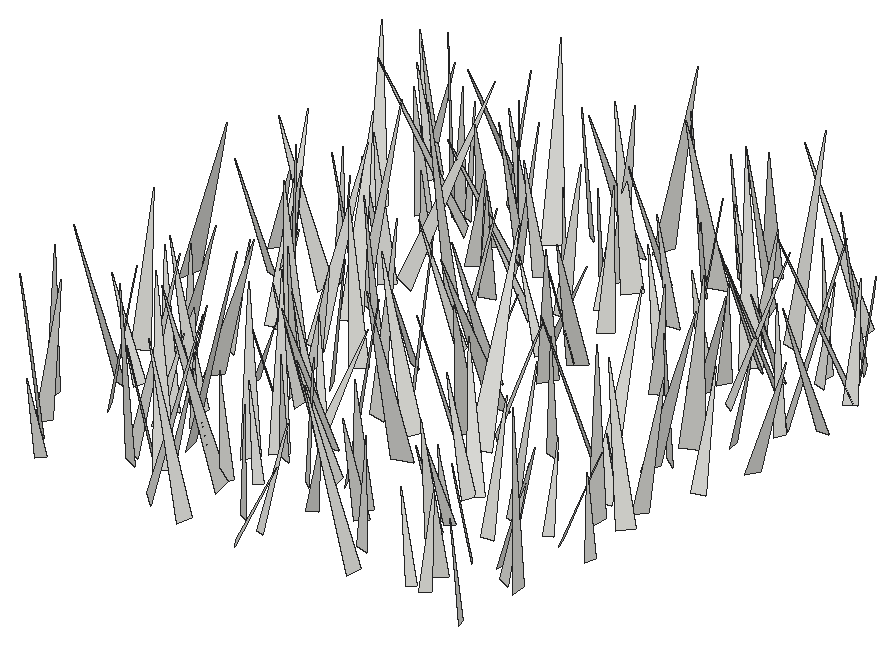
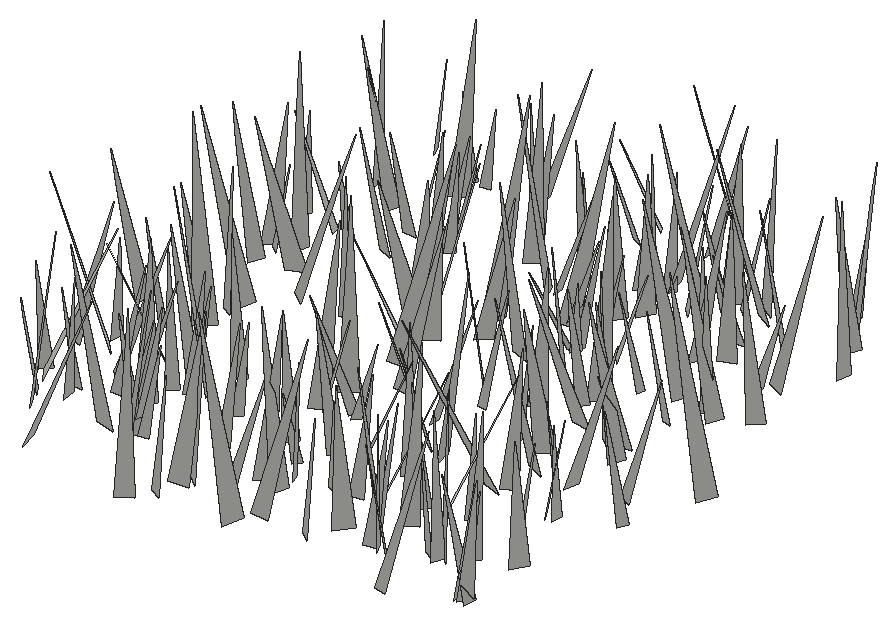
# SketchUp Ruby script. Lengths in inches.
U = 1.inch
M = Sketchup.active_model
def pt(a) = Geom::Point3d.new(a.map { |v| v * U })
def face(e, loops, mat)
  f = e.add_face(loops[0].map { |a| pt(a) })
  loops[1..].each { |l| e.add_face(l.map { |a| pt(a) }).erase! }
  f.material = f.back_material = mat if mat
  f
end
# faces: each face lists its corners as indices into pts; further lists are holes
def faces(e, pts, list, mat = nil) = list.each { |f| face(e, (f[0].is_a?(Array) ? f : [f]).map { |l| l.map { |i| pts[i] } }, mat) }
# xy, xz, yz: faces in a plane at the given z, y or x. An outline is a flat list of corners, or four numbers for a rectangle; further outlines are holes
def ring(l) = l.size == 4 ? [[l[0], l[1]], [l[2], l[1]], [l[2], l[3]], [l[0], l[3]]] : l.each_slice(2).to_a
def flat(e, list, mat, &to3) = list.each { |f| face(e, (f[0].is_a?(Array) ? f : [f]).map { |l| ring(l).map { |u, v| to3.(u, v) } }, mat) }
def xy(e, z, list, mat = nil) = flat(e, list, mat) { |x, y| [x, y, z] }
def xz(e, y, list, mat = nil) = flat(e, list, mat) { |x, z| [x, y, z] }
def yz(e, x, list, mat = nil) = flat(e, list, mat) { |y, z| [x, y, z] }
def lines(e, pts, list) = list.each { |a, b| e.add_line(pt(pts[a]), pt(pts[b])) }
# prism: a flat outline (further loops are holes) pulled along v
def prism(e, loops, v, mat = nil)
  f = face(e, loops, mat); d = Geom::Vector3d.new(v.map { |x| x * U })
  f.pushpull(f.normal.samedirection?(d) ? d.length : -d.length)
end
def box(e, o, s, mat = nil) = prism(e, [[o, [o[0] + s[0], o[1], o[2]], [o[0] + s[0], o[1] + s[1], o[2]], [o[0], o[1] + s[1], o[2]]]], [0, 0, s[2]], mat)
def at(x, y, z, deg = 0) = Geom::Transformation.translation(pt([x, y, z])) * Geom::Transformation.rotation(ORIGIN, Z_AXIS, deg.degrees)
def axes(o, x, y, z) = Geom::Transformation.new([*x, 0, *y, 0, *z, 0, *pt(o).to_a, 1])
def part(name) = M.definitions.add(name)
# library, detail: a bought-in or finely detailed component or shape, given as its bounding box
def library(name, o, s) = part(name).tap { |d| box(d.entities, o, s) }
def detail(e, o, s) = box(e.add_group.entities, o, s)
def put(e, d, t, mat = nil) = e.add_instance(d, t).tap { |i| i.material = mat if mat }
def group(e, t, mat = nil) = e.add_group.tap { |g| g.transformation = t; g.material = mat if mat }.entities
root = M.entities
c1 = part("fur_instance\#9")
p = [[0.8125,0,1.79],[0.67,-0.02,1.48],[0,-0.11,0],[0,0.11,0]]
faces(c1.entities,p,[[0,1,2,3]])
put(root,c1,axes([499.65,83.54,-21.66],[8.0282,-2.33719,0.44231],[-2.30718,-8.02996,-0.55383],[-0.57877,-0.40914,8.34313]))
put(root,c1,axes([503.88,99.4,-21.66],[-5.08982,4.44528,0.70369],[4.40622,5.13821,-0.58816],[0.91699,-0.01575,6.73207]))
put(root,c1,axes([503.84,105.55,-21.66],[3.17127,-3.30736,3.04126],[-3.82504,-3.9403,-0.2965],[-2.35731,1.94429,4.57249]))
put(root,c1,axes([501.91,90.21,-21.66],[3.6262,-2.26105,0.60128],[-2.31235,-3.63241,0.28605],[-0.35624,0.56255,4.26378]))
put(root,c1,axes([504.14,87.17,-21.66],[-1.82389,-4.57282,0.8897],[-4.65371,1.74485,-0.5721],[-0.21262,1.03617,4.88978]))
put(root,c1,axes([503.1,63.74,-21.66],[6.40054,-0.55178,2.21578],[-0.37829,-6.75939,-0.5905],[-2.25189,-0.43282,6.39709]))
put(root,c1,axes([504.66,105.33,-21.66],[-5.03296,-0.41167,1.23228],[-0.52474,5.15421,-0.42127],[1.18855,0.5323,5.03216]))
put(root,c1,axes([504.62,104.91,-21.66],[-3.50037,2.65675,1.28484],[2.86731,3.53339,0.50538],[0.69832,-1.19104,4.36526]))
put(root,c1,axes([503.78,72.875,-21.66],[3.27303,-4.65782,3.06275],[-5.40234,-3.52629,0.41046],[-1.37496,2.76738,5.67799]))
put(root,c1,axes([503.45,105.49,-21.66],[4.85484,-0.93426,0.93937],[-1.01134,-4.91828,0.33525],[-0.85583,0.51221,4.93253]))
put(root,c1,axes([505.83,68.11,-21.66],[-2.53564,-6.45433,1.27855],[-6.57975,2.48748,-0.49186],[0.00081,1.3699,6.91708]))
put(root,c1,axes([506.85,68.91,-21.66],[-3.73085,2.02538,0.45172],[2.07172,3.68874,0.57157],[0.11914,-0.71871,4.20651]))
put(root,c1,axes([504.86,60.56,-21.66],[5.24676,-2.59436,1.90695],[-2.83441,-5.4512,0.38233],[-1.5275,1.20389,5.84064]))
put(root,c1,axes([505.79,59.16,-21.66],[-4.21383,-5.23135,2.06774],[-5.35043,4.52497,0.54449],[1.7365,1.24763,6.69529]))
put(root,c1,axes([506.2,92.27,-21.66],[-3.76859,1.24193,1.36163],[1.17189,4.00702,-0.41131],[1.42236,-0.01087,3.94658]))
put(root,c1,axes([508.29,88.03,-21.66],[-6.63907,0.80935,0.83748],[0.8673,6.67065,0.42894],[0.7773,-0.53025,6.67446]))
put(root,c1,axes([507.12,92.4,-21.66],[-3.57369,-1.9669,1.0397],[-2.0892,3.64317,-0.28897],[0.76478,0.76131,4.06896]))
put(root,c1,axes([506.95,95.48,-21.66],[-3.35519,-0.75879,1.11745],[-0.66434,3.53232,0.40387],[1.17606,-0.1694,3.41613]))
put(root,c1,axes([507.09,100.62,-21.66],[4.37094,-3.26497,1.75227],[-3.26747,-4.6741,-0.55863],[-1.74761,0.57306,5.42707]))
put(root,c1,axes([507.36,73.87,-21.66],[1.49528,-4.80686,1.53266],[-5.04418,-1.45777,0.34917],[-0.10564,1.56838,5.02194]))
put(root,c1,axes([507.93,56.39,-21.66],[2.18541,-3.04998,0.78828],[-3.02604,-2.29919,-0.50659],[-0.87571,0.3334,3.71777]))
put(root,c1,axes([507.1875,65.12,-21.66],[5.44742,2.57642,1.57153],[2.74581,-5.57692,-0.37485],[-1.25227,-1.0208,6.0143]))
put(root,c1,axes([509.18,81.37,-21.66],[-1.39232,7.88876,0.40308],[7.89477,1.37627,0.33483],[-0.26016,-0.45487,8.00369]))
put(root,c1,axes([511.03,100.43,-21.66],[-6.73685,-3.71008,0.0403],[-3.70619,6.73292,0.28887],[0.17463,-0.23362,7.68547]))
put(root,c1,axes([508.9375,101.59,-21.66],[4.24793,5.0228,3.04998],[5.34423,-4.86703,0.57187],[-2.44337,-1.91294,6.55335]))
put(root,c1,axes([508.58,89.37,-21.66],[-3.28983,-1.54802,1.9149],[-2.00034,3.5437,-0.57187],[1.43591,1.38997,3.59058]))
put(root,c1,axes([506.34,74.3125,-21.66],[6.83641,-1.96558,0.32372],[-1.94381,-6.83529,-0.45298],[-0.43579,-0.34652,7.09893]))
put(root,c1,axes([508,83.29,-21.66],[5.45486,-2.53583,1.72286],[-2.73109,-5.61705,0.37948],[-1.39279,1.08278,6.00349]))
put(root,c1,axes([509.49,108.17,-21.66],[-2.17037,-5.72704,0.1674],[-5.69455,2.17595,0.61228],[0.63178,-0.0613,6.09382]))
put(root,c1,axes([509.23,81.25,-21.66],[1.43263,3.39143,0.32506],[3.34277,-1.46736,0.57677],[-0.65831,-0.07043,3.63615]))
put(root,c1,axes([508.81,76.67,-21.66],[1.57919,4.13225,1.33364],[4.34025,-1.54395,-0.35548],[-0.12772,-1.37428,4.40942]))
put(root,c1,axes([509,102.22,-21.66],[5.28351,-1.61661,1.62366],[-1.56193,-5.52709,-0.42043],[-1.67632,0.05465,5.50927]))
put(root,c1,axes([510,101.99,-21.66],[1.76175,3.91399,1.38102],[4.01071,-1.99148,0.5277],[-1.06803,-1.02224,4.25965]))
put(root,c1,axes([510.33,81.68,-21.66],[4.06784,5.47307,2.7985],[5.78633,-4.54195,0.47187],[-2.07475,-1.93641,6.80288]))
put(root,c1,axes([510.95,67.15,-21.66],[-2.98056,5.41129,1.99239],[5.72855,3.03527,0.32601],[0.65987,-1.90801,6.16924]))
put(root,c1,axes([511.4,91.1,-21.66],[-3.51075,4.42455,2.16586],[4.8357,3.60279,0.47842],[0.94002,-2.00904,5.62789]))
put(root,c1,axes([510.89,96.15,-21.66],[3.12862,-2.29976,0.97047],[-2.27,-3.26853,-0.42753],[-1.03819,0.21622,3.85932]))
put(root,c1,axes([512.72,68.39,-21.66],[-6.49588,1.72746,1.45223],[1.82521,6.62397,0.28488],[1.32729,-0.65455,6.71561]))
put(root,c1,axes([511.2,105.04,-21.66],[3.52114,3.87417,1.40413],[3.91467,-3.72163,0.45161],[-1.28689,-0.72073,5.21571]))
put(root,c1,axes([510.625,69.375,-21.66],[3.65523,2.01923,0.98653],[2.16689,-3.66612,-0.52479],[-0.59594,-0.94526,4.14277]))
put(root,c1,axes([512.76,85.38,-21.66],[-3.64093,6.72533,0.73654],[6.73348,3.68347,-0.34805],[0.65778,-0.48058,7.63972]))
put(root,c1,axes([511.72,87.85,-21.66],[2.95959,7.19025,1.54721],[7.29869,-3.07695,0.338],[-0.90704,-1.29822,7.76818]))
put(root,c1,axes([511.7,64.71,-21.66],[0.71871,3.7725,0.80138],[3.83913,-0.62217,-0.51422],[0.36739,-0.87844,3.80576]))
put(root,c1,axes([510.1,73.28,-21.66],[6.42408,-3.63909,0.41323],[-3.66082,-6.40525,0.50369],[-0.11006,0.64215,7.36601]))
put(root,c1,axes([513.28,59.77,-21.66],[2.89079,5.81329,3.19782],[6.3896,-3.37876,0.3661],[-1.787,-2.67707,6.48205]))
put(root,c1,axes([512.63,60.88,-21.66],[3.66563,6.83822,1.35122],[6.90712,-3.76874,0.33492],[-0.93742,-1.02919,7.75151]))
put(root,c1,axes([513.17,80.79,-21.66],[1.15921,7.66569,0.40932],[7.66684,-1.17697,0.3294],[-0.3873,-0.35503,7.74584]))
put(root,c1,axes([513.36,103.47,-21.66],[-4.21315,-2.34987,2.26772],[-2.4638,4.71684,0.31027],[2.14339,0.80291,4.81418]))
put(root,c1,axes([513.99,103.6,-21.66],[1.70929,-4.46495,1.67991],[-4.63149,-1.98085,-0.55231],[-1.1433,1.34907,4.74893]))
put(root,c1,axes([514.54,60.92,-21.66],[-2.99975,-3.60869,1.08185],[-3.74003,3.01886,-0.30041],[0.45307,1.02732,4.68304]))
put(root,c1,axes([512.39,91.81,-21.66],[3.274,7.7332,0.0389],[7.72076,-3.26624,-0.49451],[0.44025,-0.22856,8.38313]))
put(root,c1,axes([513.9375,66.23,-21.66],[0.22689,-3.51122,0.97081],[-3.62685,-0.12635,0.39066],[0.3422,0.98893,3.49679]))
put(root,c1,axes([512.95,74.34,-21.66],[3.6641,-0.22277,0.06955],[-0.2117,-3.63329,-0.48425],[-0.09821,-0.47926,3.63879]))
put(root,c1,axes([514.47,77.14,-21.66],[-4.81324,5.46383,3.73935],[6.29264,5.21276,0.48307],[2.05886,-3.15867,7.26549]))
put(root,c1,axes([515.17,85.24,-21.66],[-5.00491,-0.78513,1.46412],[-0.94309,5.16869,-0.45214],[1.36772,0.69095,5.0459]))
put(root,c1,axes([515.02,101.43,-21.66],[4.42222,0.57042,2.59632],[0.96066,-5.04183,-0.52855],[-2.47858,-0.93641,4.42741]))
put(root,c1,axes([513.71,99.57,-21.66],[4.30968,-5.09044,0.61484],[-5.06109,-4.35201,-0.55619],[-0.82219,0.10671,6.64655]))
put(root,c1,axes([515.89,60.39,-21.66],[-4.29093,5.93832,1.73067],[6.14946,4.32229,0.41585],[0.66564,-1.65078,7.31456]))
put(root,c1,axes([517.29,98.32,-21.66],[-5.15654,-2.89646,0.02201],[-2.88562,5.14083,0.47427],[0.2514,-0.40276,5.89529]))
put(root,c1,axes([514.44,96.9375,-21.66],[3.18493,-3.37138,0.77047],[-3.44968,-3.17103,0.3845],[-0.24394,0.82581,4.62191]))
put(root,c1,axes([514.95,78.4,-21.66],[2.82245,-3.27125,1.23973],[-3.47956,-2.78972,0.56063],[-0.36142,1.31172,4.28404]))
put(root,c1,axes([516.98,102.84,-21.66],[-5.31707,5.30249,0.96243],[5.27581,5.39738,-0.58989],[1.09932,-0.2564,7.48596]))
put(root,c1,axes([517.2,71.79,-21.66],[-2.83398,-2.56318,0.53676],[-2.6174,2.79801,-0.45803],[0.08496,0.70049,3.79362]))
put(root,c1,axes([516.24,74.73,-21.66],[5.75232,0.0292,2.58276],[0.25276,-6.28131,-0.49192],[-2.57052,-0.55229,5.73133]))
put(root,c1,axes([515.87,61.21,-21.66],[3.90442,0.1948,1.09665],[0.0575,-4.02752,0.51071],[-1.11233,0.47558,3.87577]))
put(root,c1,axes([517.37,80.45,-21.66],[-3.57367,4.96866,1.72232],[5.21894,3.60663,0.42422],[0.64547,-1.65218,6.10563]))
put(root,c1,axes([517.49,73.7,-21.66],[-4.79801,0.15244,1.14259],[0.25589,4.91001,0.4195],[1.12396,-0.46714,4.78206]))
put(root,c1,axes([517.96,90.46,-21.66],[-7.87878,-1.52664,2.20407],[-1.70967,8.13085,-0.47967],[2.06533,0.90687,8.01097]))
put(root,c1,axes([515.21,64.2,-21.66],[7.84011,2.17766,1.89393],[2.14429,-8.06482,0.39652],[-1.93163,-0.114,8.12726]))
put(root,c1,axes([517.49,63.48,-21.66],[-3.40896,-3.60182,1.17644],[-3.63778,3.55381,0.3393],[1.06005,0.61272,4.94762]))
put(root,c1,axes([516.77,99.27,-21.66],[3.29579,4.51514,1.8086],[4.80118,-3.36974,-0.33663],[-0.7786,-1.66678,5.57991]))
put(root,c1,axes([518.54,105.25,-21.66],[2.49829,3.83803,2.30798],[4.11646,-3.0089,0.54773],[-1.76409,-1.58579,4.54664]))
put(root,c1,axes([517.51,77.24,-21.66],[4.70905,2.28139,1.77217],[2.5251,-4.89691,-0.40574],[-1.40329,-1.15586,5.21682]))
put(root,c1,axes([520.57,60.99,-21.66],[-7.92829,-1.68885,1.19775],[-1.65667,8.01779,0.33921],[1.24187,-0.08605,8.09907]))
put(root,c1,axes([519.56,65.57,-21.66],[-5.3119,3.70536,1.5571],[3.75007,5.49761,-0.28937],[1.44609,-0.64586,6.4701]))
put(root,c1,axes([519.15,98.71,-21.66],[1.81609,-4.28388,1.69446],[-4.45246,-2.09973,-0.53642],[-1.18256,1.32684,4.62191]))
put(root,c1,axes([518.2,93.97,-21.66],[2.49567,-4.97649,0.70111],[-5.02561,-2.47346,0.33254],[-0.01412,0.77585,5.55727]))
put(root,c1,axes([517.63,56.43,-21.66],[5.42391,5.6075,1.42758],[5.74422,-5.4537,-0.40246],[-0.69711,-1.3092,7.79108]))
put(root,c1,axes([520.18,72.68,-21.66],[-3.13044,2.30171,0.23571],[2.28042,3.13636,-0.34054],[0.39127,0.13578,3.8706]))
put(root,c1,axes([520.18,72.33,-21.66],[-5.09295,0.86723,1.4086],[1.03106,5.23004,0.50795],[1.29351,-0.75432,5.14123]))
put(root,c1,axes([521.53,55.56,-21.66],[-6.69944,1.03913,0.45559],[1.00559,6.70154,-0.49804],[0.5255,0.42362,6.76123]))
put(root,c1,axes([520.79,67.26,-21.66],[-5.28353,4.19242,1.51467],[4.2139,5.46353,-0.42331],[1.45386,-0.59977,6.73148]))
put(root,c1,axes([519.55,89.91,-21.66],[2.50571,3.8301,0.73521],[3.84486,-2.57244,0.29737],[-0.65369,-0.44905,4.56726]))
put(root,c1,axes([521.66,86.8,-21.66],[-5.37487,-0.5228,0.79074],[-0.44432,5.41107,0.55741],[0.83736,-0.48456,5.37139]))
put(root,c1,axes([520.36,83.0625,-21.66],[-1.29347,-4.18784,0.40951],[-4.17089,1.33267,0.45438],[0.55623,0.25449,4.35943]))
put(root,c1,axes([520.32,61.89,-21.66],[3.95695,-1.9726,1.7752],[-1.97238,-4.31833,-0.40205],[-1.77544,0.40099,4.40306]))
put(root,c1,axes([522.31,93.625,-21.66],[-4.25232,-1.15186,0.17503],[-1.13335,4.24309,0.38907],[0.27009,-0.33025,4.38835]))
put(root,c1,axes([521.24,98.86,-21.66],[1.02394,3.35387,1.44831],[3.57422,-1.23084,0.32333],[-0.75567,-1.27715,3.49176]))
put(root,c1,axes([520.61,72.76,-21.66],[0.96645,3.75371,0.08435],[3.72936,-0.9496,-0.47076],[0.43512,-0.19848,3.84744]))
put(root,c1,axes([522.22,63.05,-21.66],[-1.64307,3.38565,0.94063],[3.51296,1.55882,0.52563],[-0.08077,-1.0745,3.72639]))
put(root,c1,axes([521.48,66.93,-21.66],[-0.96334,-4.21277,1.52504],[-4.43315,1.12201,0.29911],[0.64835,1.41239,4.31115]))
put(root,c1,axes([522.96,69.56,-21.66],[-3.66432,1.46778,0.50332],[1.5223,3.65057,0.437],[0.30055,-0.59495,3.9231]))
put(root,c1,axes([522.8,105.125,-21.66],[-0.03159,-6.8611,0.78211],[-6.88005,-0.03586,-0.59249],[-0.59273,0.78192,6.83555]))
put(root,c1,axes([522.4375,80.28,-21.66],[-3.91577,-3.49387,3.17429],[-4.26524,4.38586,-0.43413],[2.02262,2.48468,5.2299]))
put(root,c1,axes([522.86,75.64,-21.66],[2.04699,7.14679,2.15899],[7.40344,-2.23185,0.36858],[-0.96272,-1.9673,7.42502]))
put(root,c1,axes([522.91,70.1,-21.66],[1.39715,-7.46285,0.32526],[-7.45597,-1.41344,-0.40331],[-0.45656,0.24497,7.58179]))
put(root,c1,axes([524.45,58.59,-21.66],[2.05844,3.54151,1.67651],[3.74882,-2.33096,0.32115],[-1.13989,-1.27062,4.08367]))
put(root,c1,axes([524.21,99.33,-21.66],[-3.74193,-1.93414,1.83822],[-1.95383,4.14237,0.38123],[1.81727,0.47108,4.19495]))
put(root,c1,axes([523.98,95.07,-21.66],[-0.55684,5.82392,2.02647],[6.12632,0.75415,-0.48394],[0.70204,-1.96161,5.83043]))
put(root,c1,axes([526.38,75.29,-21.66],[-5.76808,3.66085,1.08427],[3.77252,5.76709,0.59739],[0.58783,-1.08949,6.80556]))
put(root,c1,axes([523.99,101.35,-21.66],[6.73151,-1.98165,2.55494],[-2.23492,-7.11595,0.36912],[-2.33662,1.09735,7.00742]))
put(root,c1,axes([525.8125,100.8,-21.66],[-4.89648,5.17695,2.06152],[5.4889,4.95404,0.59637],[0.96057,-1.91907,7.10075]))
put(root,c1,axes([525.01,65.1,-21.66],[2.79154,3.79561,1.789],[3.98615,-3.06992,0.29332],[-1.31064,-1.25251,4.70248]))
put(root,c1,axes([526.23,89.9,-21.66],[-3.21224,1.96871,0.46482],[2.01704,3.18335,0.45637],[0.15311,-0.63315,3.7398]))
put(root,c1,axes([526.51,66.79,-21.66],[-4.93591,-0.64757,0.62999],[-0.58328,4.95621,0.52453],[0.68994,-0.44273,4.95049]))
put(root,c1,axes([523.76,106.9,-21.66],[7.67247,-2.21843,2.0813],[-2.41925,-7.8734,0.52613],[-1.84403,1.09916,7.96941]))
put(root,c1,axes([525.47,97.43,-21.66],[-2.23531,2.8422,0.49749],[2.78374,2.28983,-0.57415],[0.75919,-0.0278,3.57002]))
put(root,c1,axes([526.15,84.84,-21.66],[-0.27695,-6.43694,1.01641],[-6.49492,0.18954,-0.56932],[-0.53231,1.03627,6.4177]))
put(root,c1,axes([526.73,103.57,-21.66],[-1.73362,-4.79917,0.85478],[-4.86621,1.65027,-0.60395],[-0.28757,1.00633,5.06683]))
put(root,c1,axes([525.11,84.91,-21.66],[2.99336,2.37967,0.42143],[2.41657,-2.95437,-0.48225],[-0.02533,-0.63994,3.79348]))
put(root,c1,axes([526.73,57.6,-21.66],[1.45638,3.8911,0.37542],[3.87774,-1.48869,0.38679],[-0.49475,-0.21394,4.13668]))
put(root,c1,axes([527.8,95.32,-21.66],[3.60386,-3.42869,2.87422],[-4.08632,-4.02533,0.32181],[-1.82182,2.24626,4.96388]))
put(root,c1,axes([528.625,90.61,-21.66],[-2.84095,-2.72325,0.75235],[-2.80656,2.8428,-0.30791],[0.32453,0.74533,3.9233]))
put(root,c1,axes([526.33,55.36,-21.66],[3.11612,2.14822,0.04863],[2.13222,-3.08072,-0.53874],[0.26618,-0.47091,3.74631]))
put(root,c1,axes([526.97,67.23,-21.66],[6.97385,3.06548,2.09729],[3.25235,-7.19468,-0.2986],[-1.79388,-1.12684,7.61201]))
put(root,c1,axes([528.1,71.95,-21.66],[1.76512,-7.95634,1.31885],[-8.03843,-1.84494,-0.37166],[-0.65291,1.20466,8.14131]))
put(root,c1,axes([526.91,89.29,-21.66],[4.6922,-0.3007,0.23761],[-0.32477,-4.66947,0.50417],[-0.20347,0.51889,4.67471]))
put(root,c1,axes([528.875,81.96,-21.66],[0.62863,-8.27068,0.12443],[-8.26435,-0.63324,-0.33804],[-0.34653,0.09834,8.28764]))
put(root,c1,axes([527.71,62.3,-21.66],[2.72527,-3.47225,0.02549],[-3.46346,-2.7159,0.33551],[0.24824,0.22715,4.40125]))
put(root,c1,axes([529.75,103.93,-21.66],[-4.37552,-5.12362,2.64469],[-5.63456,4.50416,-0.59611],[1.22377,2.41912,6.71129]))
put(root,c1,axes([530.19,105.03,-21.66],[1.08245,-7.41016,1.80762],[-7.58562,-1.23679,-0.52762],[-0.7977,1.70574,7.47019]))
put(root,c1,axes([530.59,107.07,-21.66],[1.70203,4.17643,2.24286],[4.55719,-2.09788,0.44817],[-1.30578,-1.87783,4.48761]))
put(root,c1,axes([531.12,74.9375,-21.66],[-4.99483,-3.69291,1.05885],[-3.66459,5.10128,0.50484],[1.15306,0.21561,6.19121]))
put(root,c1,axes([529.18,90.41,-21.66],[3.47226,-5.91321,0.27335],[-5.89868,-3.48291,-0.41506],[-0.49636,0.02495,6.84473]))
put(root,c1,axes([529.03,87.21,-21.66],[5.34448,-4.72432,0.68412],[-4.69665,-5.3877,-0.51471],[-0.85369,0.0645,7.11462]))
put(root,c1,axes([531.41,76.55,-21.66],[-2.88963,7.72101,0.14725],[7.7077,2.8933,-0.45358],[0.4764,0.02131,8.23153]))
put(root,c1,axes([529.3,77.78,-21.66],[4.72004,-5.82808,0.22381],[-5.80637,-4.72269,-0.52693],[-0.55017,-0.15829,7.48115]))
put(root,c1,axes([531.09,98.81,-21.66],[0.46643,-4.66615,1.44002],[-4.86096,-0.58186,-0.31092],[-0.46655,1.39737,4.67909]))
put(root,c1,axes([530.48,64.55,-21.66],[4.51111,-4.76568,1.07484],[-4.75985,-4.61702,-0.49408],[-1.1004,0.43419,6.54353]))
put(root,c1,axes([531.24,63.47,-21.66],[2.7716,-4.32676,0.73791],[-4.29866,-2.85215,-0.57784],[-0.88707,0.30254,5.10575]))
put(root,c1,axes([531.25,78.64,-21.66],[3.44436,3.22324,0.28553],[3.18394,-3.45028,0.54084],[-0.57733,0.20181,4.68619]))
put(root,c1,axes([533.06,94.79,-21.66],[-3.14224,2.77876,1.0294],[2.91205,3.17344,0.32264],[0.54877,-0.92877,4.18224]))
put(root,c1,axes([535.43,57.3,-21.66],[-7.05219,-0.0174,0.36445],[-0.04272,7.04446,-0.49029],[0.36236,0.49184,7.03515]))
put(root,c1,axes([531.95,108.875,-21.66],[2.97455,-6.14482,0.55918],[-6.16848,-2.94679,0.43089],[0.14598,0.69067,6.8133]))
put(root,c1,axes([535.46,71.03,-21.66],[-3.60755,4.52257,0.00535],[4.517,3.60276,0.29145],[-0.22451,-0.18592,5.77782]))
put(root,c1,axes([535.18,70.63,-21.66],[-4.286,2.05614,0.85108],[2.13965,4.31523,0.34994],[0.6115,-0.68765,4.74078]))
put(root,c1,axes([533.83,60.22,-21.66],[0.99186,4.25892,2.03749],[4.71935,-0.95274,-0.30591],[-0.13232,-2.05608,4.36218]))
put(root,c1,axes([535.16,104.82,-21.66],[-6.26815,-2.22604,2.13273],[-2.17784,6.6177,0.5065],[2.18193,0.21043,6.63238]))
put(root,c1,axes([536.3,101.29,-21.66],[0.92533,-3.44435,1.34936],[-3.58141,-1.18238,-0.56215],[-0.92618,1.13092,3.52189]))
put(root,c1,axes([536.99,100.79,-21.66],[-4.76846,2.17787,1.48985],[2.383,4.8757,0.4998],[1.13316,-1.08876,5.21838]))
put(root,c1,axes([536.02,67.08,-21.66],[2.32734,-2.83374,0.7234],[-2.82694,-2.41664,-0.37171],[-0.74954,0.31569,3.64807]))
put(root,c1,axes([536.98,65.13,-21.66],[-3.57828,-1.18752,0.86435],[-1.11493,3.67791,0.43741],[0.95617,-0.15551,3.74473]))
put(root,c1,axes([535.97,79.01,-21.66],[-0.76363,-5.08076,1.72351],[-5.30047,0.98391,0.55201],[0.83046,1.60796,5.10809]))
put(root,c1,axes([536.47,66.84,-21.66],[1.6071,-3.85332,0.26864],[-3.82652,-1.62792,-0.45895],[-0.52725,0.06941,4.14972]))
put(root,c1,axes([536.24,90.53,-21.66],[2.86346,-4.49186,1.0378],[-4.60706,-2.8331,0.44926],[-0.16992,1.11803,5.30796]))
put(root,c1,axes([537.66,94.32,-21.66],[-3.6167,2.28369,2.19841],[2.80718,3.85669,0.61192],[1.47241,-1.74341,4.23336]))
put(root,c1,axes([536.8125,101.24,-21.66],[4.06657,-2.17936,1.39694],[-2.40276,-4.14574,0.52683],[-0.9632,1.14071,4.58356]))
put(root,c1,axes([539.01,97.61,-21.66],[-6.71454,4.39928,1.56364],[4.39375,6.8803,-0.4901],[1.57912,-0.43767,8.0124]))
put(root,c1,axes([538.4,100.43,-21.66],[-1.63509,-3.83691,0.93062],[-3.94815,1.58786,-0.39017],[-0.00453,1.00909,4.15248]))
put(root,c1,axes([536.8125,93.39,-21.66],[7.03431,3.48518,2.0857],[3.73576,-7.18871,-0.58711],[-1.59396,-1.46769,7.82836]))
put(root,c1,axes([539.73,97.79,-21.66],[-2.91722,-4.26379,0.81225],[-4.33997,2.88016,-0.46811],[0.06569,0.93518,5.14499]))
put(root,c1,axes([540.28,78.9,-21.66],[-3.80657,-5.75041,0.9295],[-5.82495,3.76407,-0.56819],[0.03325,1.08891,6.87272]))
put(root,c1,axes([539.85,58.3125,-21.66],[-1.79664,3.17113,0.9039],[3.29721,1.71578,0.53432],[-0.03822,-1.04932,3.60534]))
put(root,c1,axes([542.33,106.74,-21.66],[-7.29173,-1.24054,0.1592],[-1.24954,7.26646,-0.60898],[0.05425,0.6271,7.37139]))
put(root,c1,axes([539.83,66.875,-21.66],[0.07202,5.27236,0.64208],[5.29211,-0.12578,0.43929],[-0.45123,-0.63374,5.25452]))
put(root,c1,axes([539.5625,70.03,-21.66],[1.82838,5.64567,1.15342],[5.69001,-1.95997,0.57384],[-0.90985,-0.91206,5.90655]))
put(root,c1,axes([539.45,101.75,-21.66],[1.82525,7.99707,1.79582],[8.16577,-1.93273,0.30716],[-0.70587,-1.67961,8.19697]))
put(root,c1,axes([538.95,94.73,-21.66],[4.27597,-2.96302,0.67606],[-2.94629,-4.32773,-0.33261],[-0.74558,0.10858,5.19161]))
put(root,c1,axes([541,63.72,-21.66],[-2.98198,-2.20876,0.85448],[-2.34628,2.94214,-0.58291],[0.32208,0.98295,3.66484]))
put(root,c1,axes([540.54,60.43,-21.66],[3.54462,-5.56954,2.15269],[-5.7416,-3.86654,-0.54956],[-1.63946,1.49942,6.57891]))
put(root,c1,axes([538.67,92.62,-21.66],[5.31861,-1.95589,0.12332],[-1.94358,-5.30997,-0.39374],[-0.25139,-0.32717,5.65315]))
put(root,c1,axes([541.16,58.22,-21.66],[-2.54986,2.80817,1.27437],[2.87177,2.76487,-0.34653],[1.12374,-0.69377,3.77724]))
put(root,c1,axes([541.75,97.62,-21.66],[-0.76321,-4.71965,0.1503],[-4.6984,0.77422,0.45372],[0.47201,0.07524,4.75939]))
put(root,c1,axes([543.2,95.64,-21.66],[-2.96525,-5.05492,0.58848],[-5.08807,2.93137,-0.45808],[-0.10025,0.73898,5.84252]))
put(root,c1,axes([541.26,92.32,-21.66],[3.77289,4.9439,0.17652],[4.9129,-3.7705,0.5956],[-0.58026,0.22179,6.19049]))
put(root,c1,axes([542.8125,75.89,-21.66],[-2.31741,7.72302,0.72504],[7.71845,2.37113,-0.58682],[0.77216,-0.52327,8.04183]))
put(root,c1,axes([542.9375,69.89,-21.66],[-2.61192,2.51011,0.78878],[2.46687,2.72278,-0.49597],[0.91509,-0.17543,3.58843]))
put(root,c1,axes([543.04,83.49,-21.66],[-2.5079,-4.6968,1.95628],[-4.90602,2.8103,0.45782],[1.34828,1.48955,5.3047]))
put(root,c1,axes([544.18,99.91,-21.66],[-5.10853,0.04095,1.59169],[-0.11644,5.32521,-0.51071],[1.58796,0.52222,5.08311]))
put(root,c1,axes([542.99,86.01,-21.66],[4.39252,-6.51911,2.0007],[-6.79057,-4.39945,0.57342],[-0.62428,1.98542,7.83991]))
put(root,c1,axes([542.5,82,-21.66],[7.35605,-1.97253,1.00478],[-2.03855,-7.39535,0.40615],[-0.86301,0.65556,7.60509]))
put(root,c1,axes([544.4,98.63,-21.66],[0.69151,3.97199,1.28395],[4.17346,-0.6309,-0.296],[0.08642,-1.31479,4.02085]))
put(root,c1,axes([544.48,73.45,-21.66],[7.21029,-1.27081,2.71678],[-1.16788,-7.70491,-0.50453],[-2.76259,-0.05954,7.30402]))
put(root,c1,axes([547.45,98.67,-21.66],[-5.40162,-4.18627,0.13743],[-4.18531,5.38577,-0.4449],[-0.16419,0.43574,6.81941]))
put(root,c1,axes([545.53,102.36,-21.66],[-5.52938,-3.456,2.07939],[-3.45701,5.87854,0.57763],[2.07771,0.58365,6.49494]))
put(root,c1,axes([543.05,64.75,-21.66],[6.29896,-1.22347,0.37639],[-1.1888,-6.29213,-0.55798],[-0.47466,-0.47719,6.39237]))
put(root,c1,axes([545.92,56.29,-21.66],[-3.70453,-1.18645,1.17686],[-1.32576,3.8289,-0.31316],[1.01735,0.66938,3.87726]))
put(root,c1,axes([545.98,74.4,-21.66],[-2.17091,-2.72609,1.07786],[-2.90812,2.17161,-0.36485],[0.36901,1.07644,3.46573]))
put(root,c1,axes([546.6,74.02,-21.66],[-4.49758,4.50366,1.60112],[4.72062,4.53017,0.51777],[0.74986,-1.50644,6.34374]))
put(root,c1,axes([544.67,62.72,-21.66],[2.00613,4.44684,1.43472],[4.67253,-1.91449,-0.59961],[-0.01581,-1.5549,4.84142]))
put(root,c1,axes([546.21,62.4375,-21.66],[-6.67663,-0.80436,2.4344],[-1.05353,7.05179,-0.55944],[2.33738,0.88086,6.7016]))
put(root,c1,axes([546.67,91.33,-21.66],[-4.5869,1.43943,1.05541],[1.33614,4.69877,-0.60151],[1.18347,0.27406,4.76967]))
put(root,c1,axes([545,88.18,-21.66],[4.1341,0.32333,0.78637],[0.3951,-4.18703,-0.35553],[-0.75288,-0.42186,4.13146]))
put(root,c1,axes([544.1875,69.74,-21.66],[4.46845,1.48023,0.19389],[1.49287,-4.43008,-0.58427],[0.00126,-0.6156,4.67084]))
put(root,c1,axes([546.32,100.75,-21.66],[3.3556,2.16226,1.21696],[2.08771,-3.56664,0.58052],[-1.34083,-0.14202,3.94948]))
put(root,c1,axes([546,76.43,-21.66],[5.31281,-2.73186,1.51927],[-2.91837,-5.40827,0.48055],[-1.11999,1.13346,5.95467]))
put(root,c1,axes([547.43,81.18,-21.66],[-2.09366,4.25191,0.8072],[4.26644,2.17826,-0.40798],[0.72654,-0.53866,4.72184]))
put(root,c1,axes([546.2,92.75,-21.66],[5.62974,5.25868,1.12192],[5.27805,-5.71471,0.30107],[-1.02693,-0.54292,7.69786]))
put(root,c1,axes([547.47,68.98,-21.66],[3.35457,-1.66316,1.27005],[-1.64462,-3.57909,-0.343],[-1.29397,0.23728,3.72849]))
put(root,c1,axes([547.81,97.83,-21.66],[-2.87037,3.7349,1.34525],[3.80013,3.06525,-0.40189],[1.14815,-0.80807,4.69329]))
put(root,c1,axes([548.74,93.58,-21.66],[-0.82643,-5.48525,0.94931],[-5.54864,0.73423,-0.58792],[-0.44918,1.02229,5.51591]))
put(root,c1,axes([548.5625,85.96,-21.66],[5.12871,-2.48578,0.55768],[-2.53054,-5.11559,0.47007],[-0.29413,0.66743,5.67995]))
